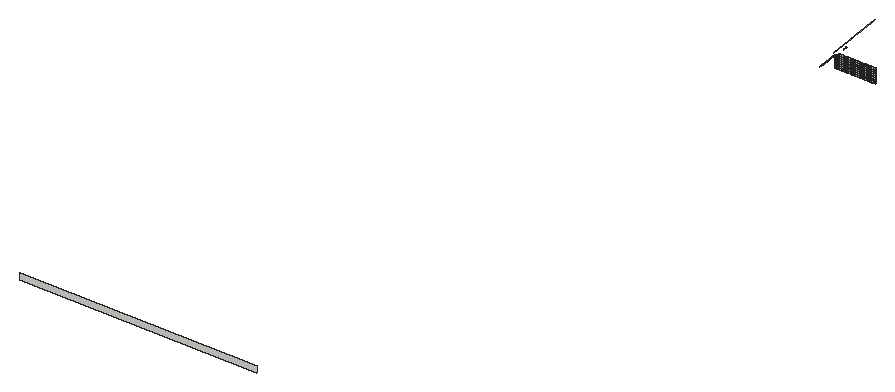
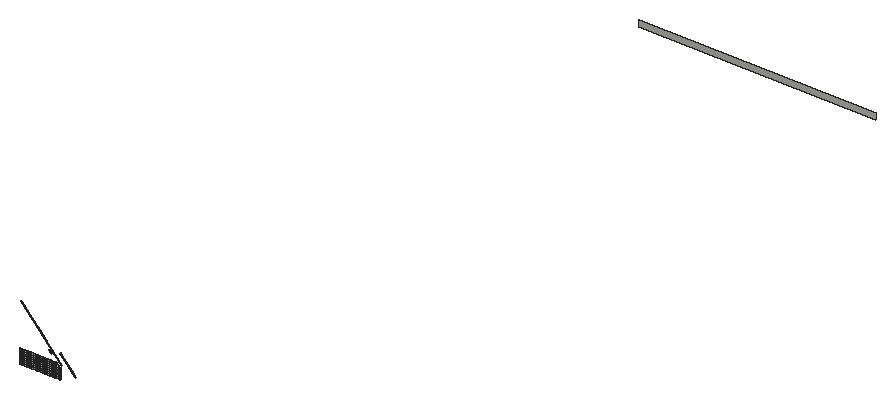
# SketchUp Ruby script. Lengths in inches.
U = 1.inch
M = Sketchup.active_model
def pt(a) = Geom::Point3d.new(a.map { |v| v * U })
def face(e, loops, mat)
  f = e.add_face(loops[0].map { |a| pt(a) })
  loops[1..].each { |l| e.add_face(l.map { |a| pt(a) }).erase! }
  f.material = f.back_material = mat if mat
  f
end
# faces: each face lists its corners as indices into pts; further lists are holes
def faces(e, pts, list, mat = nil) = list.each { |f| face(e, (f[0].is_a?(Array) ? f : [f]).map { |l| l.map { |i| pts[i] } }, mat) }
# xy, xz, yz: faces in a plane at the given z, y or x. An outline is a flat list of corners, or four numbers for a rectangle; further outlines are holes
def ring(l) = l.size == 4 ? [[l[0], l[1]], [l[2], l[1]], [l[2], l[3]], [l[0], l[3]]] : l.each_slice(2).to_a
def flat(e, list, mat, &to3) = list.each { |f| face(e, (f[0].is_a?(Array) ? f : [f]).map { |l| ring(l).map { |u, v| to3.(u, v) } }, mat) }
def xy(e, z, list, mat = nil) = flat(e, list, mat) { |x, y| [x, y, z] }
def xz(e, y, list, mat = nil) = flat(e, list, mat) { |x, z| [x, y, z] }
def yz(e, x, list, mat = nil) = flat(e, list, mat) { |y, z| [x, y, z] }
def lines(e, pts, list) = list.each { |a, b| e.add_line(pt(pts[a]), pt(pts[b])) }
# prism: a flat outline (further loops are holes) pulled along v
def prism(e, loops, v, mat = nil)
  f = face(e, loops, mat); d = Geom::Vector3d.new(v.map { |x| x * U })
  f.pushpull(f.normal.samedirection?(d) ? d.length : -d.length)
end
def box(e, o, s, mat = nil) = prism(e, [[o, [o[0] + s[0], o[1], o[2]], [o[0] + s[0], o[1] + s[1], o[2]], [o[0], o[1] + s[1], o[2]]]], [0, 0, s[2]], mat)
def at(x, y, z, deg = 0) = Geom::Transformation.translation(pt([x, y, z])) * Geom::Transformation.rotation(ORIGIN, Z_AXIS, deg.degrees)
def axes(o, x, y, z) = Geom::Transformation.new([*x, 0, *y, 0, *z, 0, *pt(o).to_a, 1])
def part(name) = M.definitions.add(name)
# library, detail: a bought-in or finely detailed component or shape, given as its bounding box
def library(name, o, s) = part(name).tap { |d| box(d.entities, o, s) }
def detail(e, o, s) = box(e.add_group.entities, o, s)
def put(e, d, t, mat = nil) = e.add_instance(d, t).tap { |i| i.material = mat if mat }
def group(e, t, mat = nil) = e.add_group.tap { |g| g.transformation = t; g.material = mat if mat }.entities
root = M.entities
M.materials.add("[Color M06]").color = [79, 71, 84]
xy(root,305.35,[[951.9,2332.13,954.21,2332.76],[954.8125,2332.13,957.125,2332.76],[957.72,2332.13,960.04,2332.76],[960.64,2332.13,962.95,2332.76],[963.55,2332.13,965.86,2332.76],
  [966.46,2332.13,968.77,2332.76],[969.375,2332.13,971.6875,2332.76],[972.29,2332.13,974.6,2332.76],[975.2,2332.13,977.51,2332.76],[978.11,2332.13,980.42,2332.76],
  [981.02,2332.13,983.33,2332.76],[983.93,2332.13,986.25,2332.76],[986.85,2332.13,989.16,2332.76],[989.76,2332.13,992.07,2332.76],[992.67,2332.13,994.98,2332.76],
  [995.58,2332.13,997.89,2332.76],[998.49,2332.13,1000.81,2332.63],[1001.41,2332.13,1003.72,2332.63],[1004.32,2332.13,1006.63,2332.63],[1007.23,2332.13,1009.54,2332.63],
  [1010.14,2332.13,1012.45,2332.76],[1013.05,2332.13,1015.37,2332.76],[1015.97,2332.13,1018.28,2332.76]])
xy(root,307.67,[[951.9,2332.13,954.21,2332.76],[954.8125,2332.13,957.125,2332.76],[957.72,2332.13,960.04,2332.76],[960.64,2332.13,962.95,2332.76],[963.55,2332.13,965.86,2332.76],
  [966.46,2332.13,968.77,2332.76],[969.375,2332.13,971.6875,2332.76],[972.29,2332.13,974.6,2332.76],[975.2,2332.13,977.51,2332.76],[978.11,2332.13,980.42,2332.76],
  [981.02,2332.13,983.33,2332.76],[983.93,2332.13,986.25,2332.76],[986.85,2332.13,989.16,2332.76],[989.76,2332.13,992.07,2332.76],[992.67,2332.13,994.98,2332.76],
  [995.58,2332.13,997.89,2332.76],[998.49,2332.13,1000.81,2332.63],[1001.41,2332.13,1003.72,2332.63],[1004.32,2332.13,1006.63,2332.63],[1007.23,2332.13,1009.54,2332.63],
  [1010.14,2332.13,1012.45,2332.76],[1013.05,2332.13,1015.37,2332.76],[1015.97,2332.13,1018.28,2332.76]])
xy(root,308.4,[[951.93,2332.13,954.24,2332.76],[954.84,2332.13,957.15,2332.76],[957.75,2332.13,960.07,2332.76],[960.67,2332.13,962.98,2332.76],[963.58,2332.13,965.89,2332.76],
  [966.49,2332.13,968.8,2332.76],[969.4,2332.13,971.71,2332.76],[972.3125,2332.13,974.625,2332.76],[975.23,2332.13,977.54,2332.76],[978.14,2332.13,980.45,2332.76],
  [981.05,2332.13,983.36,2332.76],[983.96,2332.13,986.27,2332.76],[986.875,2332.13,989.1875,2332.76],[989.79,2332.13,992.1,2332.76],[992.7,2332.13,995.01,2332.76],
  [995.61,2332.13,997.92,2332.76],[998.52,2332.13,1000.83,2332.76],[1001.43,2332.13,1003.75,2332.76],[1004.35,2332.13,1006.66,2332.76],[1007.26,2332.13,1009.57,2332.76],
  [1010.17,2332.13,1012.48,2332.76],[1013.08,2332.13,1015.4,2332.76],[1015.99,2332.13,1018.31,2332.76]])
xy(root,310.71,[[951.93,2332.13,954.24,2332.76],[954.84,2332.13,957.15,2332.76],[957.75,2332.13,960.07,2332.76],[960.67,2332.13,962.98,2332.76],[963.58,2332.13,965.89,2332.76],
  [966.49,2332.13,968.8,2332.76],[969.4,2332.13,971.71,2332.76],[972.3125,2332.13,974.625,2332.76],[975.23,2332.13,977.54,2332.76],[978.14,2332.13,980.45,2332.76],
  [981.05,2332.13,983.36,2332.76],[983.96,2332.13,986.27,2332.76],[986.875,2332.13,989.1875,2332.76],[989.79,2332.13,992.1,2332.76],[992.7,2332.13,995.01,2332.76],
  [995.61,2332.13,997.92,2332.76],[998.52,2332.13,1000.83,2332.76],[1001.43,2332.13,1003.75,2332.76],[1004.35,2332.13,1006.66,2332.76],[1007.26,2332.13,1009.57,2332.76],
  [1010.17,2332.13,1012.48,2332.76],[1013.08,2332.13,1015.4,2332.76],[1015.99,2332.13,1018.31,2332.76]])
xy(root,311.21,[[951.93,2332.13,954.24,2332.76],[954.84,2332.13,957.15,2332.76],[957.75,2332.13,960.07,2332.76],[960.67,2332.13,962.98,2332.76],[963.58,2332.13,965.89,2332.76],
  [966.49,2332.13,968.8,2332.76],[969.4,2332.13,971.71,2332.76],[972.3125,2332.13,974.625,2332.76],[975.23,2332.13,977.54,2332.76],[978.14,2332.13,980.45,2332.76],
  [981.05,2332.13,983.36,2332.76],[983.96,2332.13,986.27,2332.76],[986.875,2332.13,989.1875,2332.76],[989.79,2332.13,992.1,2332.76],[992.7,2332.13,995.01,2332.76],
  [995.61,2332.13,997.92,2332.76],[998.52,2332.13,1000.83,2332.76],[1001.43,2332.13,1003.75,2332.76],[1004.35,2332.13,1006.66,2332.76],[1007.26,2332.13,1009.57,2332.76],
  [1010.17,2332.13,1012.48,2332.76],[1013.08,2332.13,1015.4,2332.76],[1015.99,2332.13,1018.31,2332.76]])
xy(root,313.52,[[951.93,2332.13,954.24,2332.76],[954.84,2332.13,957.15,2332.76],[957.75,2332.13,960.07,2332.76],[960.67,2332.13,962.98,2332.76],[963.58,2332.13,965.89,2332.76],
  [966.49,2332.13,968.8,2332.76],[969.4,2332.13,971.71,2332.76],[972.3125,2332.13,974.625,2332.76],[975.23,2332.13,977.54,2332.76],[978.14,2332.13,980.45,2332.76],
  [981.05,2332.13,983.36,2332.76],[983.96,2332.13,986.27,2332.76],[986.875,2332.13,989.1875,2332.76],[989.79,2332.13,992.1,2332.76],[992.7,2332.13,995.01,2332.76],
  [995.61,2332.13,997.92,2332.76],[998.52,2332.13,1000.83,2332.76],[1001.43,2332.13,1003.75,2332.76],[1004.35,2332.13,1006.66,2332.76],[1007.26,2332.13,1009.57,2332.76],
  [1010.17,2332.13,1012.48,2332.76],[1013.08,2332.13,1015.4,2332.76],[1015.99,2332.13,1018.31,2332.76]])
xy(root,314.02,[[951.93,2332.13,954.24,2332.76],[954.84,2332.13,957.15,2332.76],[957.75,2332.13,960.07,2332.76],[960.67,2332.13,962.98,2332.76],[963.58,2332.13,965.89,2332.76],
  [966.49,2332.13,968.8,2332.76],[969.4,2332.13,971.71,2332.76],[972.3125,2332.13,974.625,2332.76],[975.23,2332.13,977.54,2332.76],[978.14,2332.13,980.45,2332.76],
  [981.05,2332.13,983.36,2332.76],[983.96,2332.13,986.27,2332.76],[986.875,2332.13,989.1875,2332.76],[989.79,2332.13,992.1,2332.76],[992.7,2332.13,995.01,2332.76],
  [995.61,2332.13,997.92,2332.76],[998.52,2332.13,1000.83,2332.76],[1001.43,2332.13,1003.75,2332.76],[1004.35,2332.13,1006.66,2332.76],[1007.26,2332.13,1009.57,2332.76],
  [1010.17,2332.13,1012.48,2332.76],[1013.08,2332.13,1015.4,2332.76],[1015.99,2332.13,1018.31,2332.76]])
xy(root,316.34,[[951.93,2332.13,954.24,2332.76],[954.84,2332.13,957.15,2332.76],[957.75,2332.13,960.07,2332.76],[960.67,2332.13,962.98,2332.76],[963.58,2332.13,965.89,2332.76],
  [966.49,2332.13,968.8,2332.76],[969.4,2332.13,971.71,2332.76],[972.3125,2332.13,974.625,2332.76],[975.23,2332.13,977.54,2332.76],[978.14,2332.13,980.45,2332.76],
  [981.05,2332.13,983.36,2332.76],[983.96,2332.13,986.27,2332.76],[986.875,2332.13,989.1875,2332.76],[989.79,2332.13,992.1,2332.76],[992.7,2332.13,995.01,2332.76],
  [995.61,2332.13,997.92,2332.76],[998.52,2332.13,1000.83,2332.76],[1001.43,2332.13,1003.75,2332.76],[1004.35,2332.13,1006.66,2332.76],[1007.26,2332.13,1009.57,2332.76],
  [1010.17,2332.13,1012.48,2332.76],[1013.08,2332.13,1015.4,2332.76],[1015.99,2332.13,1018.31,2332.76]])
xy(root,316.84,[[951.93,2332.13,954.24,2332.76],[954.84,2332.13,957.15,2332.76],[957.75,2332.13,960.07,2332.76],[960.67,2332.13,962.98,2332.76],[963.58,2332.13,965.89,2332.76],
  [966.49,2332.13,968.8,2332.76],[969.4,2332.13,971.71,2332.76],[972.3125,2332.13,974.625,2332.76],[975.23,2332.13,977.54,2332.76],[978.14,2332.13,980.45,2332.76],
  [981.05,2332.13,983.36,2332.76],[983.96,2332.13,986.27,2332.76],[986.875,2332.13,989.1875,2332.76],[989.79,2332.13,992.1,2332.76],[992.7,2332.13,995.01,2332.76],
  [995.61,2332.13,997.92,2332.76],[998.52,2332.13,1000.83,2332.76],[1001.43,2332.13,1003.75,2332.76],[1004.35,2332.13,1006.66,2332.76],[1007.26,2332.13,1009.57,2332.76],
  [1010.17,2332.13,1012.48,2332.76],[1013.08,2332.13,1015.4,2332.76],[1015.99,2332.13,1018.31,2332.76]])
xy(root,319.15,[[951.93,2332.13,954.24,2332.76],[954.84,2332.13,957.15,2332.76],[957.75,2332.13,960.07,2332.76],[960.67,2332.13,962.98,2332.76],[963.58,2332.13,965.89,2332.76],
  [966.49,2332.13,968.8,2332.76],[969.4,2332.13,971.71,2332.76],[972.3125,2332.13,974.625,2332.76],[975.23,2332.13,977.54,2332.76],[978.14,2332.13,980.45,2332.76],
  [981.05,2332.13,983.36,2332.76],[983.96,2332.13,986.27,2332.76],[986.875,2332.13,989.1875,2332.76],[989.79,2332.13,992.1,2332.76],[992.7,2332.13,995.01,2332.76],
  [995.61,2332.13,997.92,2332.76],[998.52,2332.13,1000.83,2332.76],[1001.43,2332.13,1003.75,2332.76],[1004.35,2332.13,1006.66,2332.76],[1007.26,2332.13,1009.57,2332.76],
  [1010.17,2332.13,1012.48,2332.76],[1013.08,2332.13,1015.4,2332.76],[1015.99,2332.13,1018.31,2332.76]])
xy(root,319.65,[[951.93,2332.13,954.24,2332.76],[954.84,2332.13,957.15,2332.76],[957.75,2332.13,960.07,2332.76],[960.67,2332.13,962.98,2332.76],[963.58,2332.13,965.89,2332.76],
  [966.49,2332.13,968.8,2332.76],[969.4,2332.13,971.71,2332.76],[972.3125,2332.13,974.625,2332.76],[975.23,2332.13,977.54,2332.76],[978.14,2332.13,980.45,2332.76],
  [981.05,2332.13,983.36,2332.76],[983.96,2332.13,986.27,2332.76],[986.875,2332.13,989.1875,2332.76],[989.79,2332.13,992.1,2332.76],[992.7,2332.13,995.01,2332.76],
  [995.61,2332.13,997.92,2332.76],[998.52,2332.13,1000.83,2332.76],[1001.43,2332.13,1003.75,2332.76],[1004.35,2332.13,1006.66,2332.7],[1007.26,2332.13,1009.57,2332.7],
  [1010.17,2332.13,1012.48,2332.7],[1013.08,2332.13,1015.4,2332.7],[1015.99,2332.13,1018.31,2332.76]])
xy(root,321.96,[[952.46,2332.13,954.24,2332.76],[954.84,2332.13,957.15,2332.76],[957.75,2332.13,960.07,2332.76],[960.67,2332.13,962.98,2332.76],[963.58,2332.13,965.89,2332.76],
  [966.49,2332.13,968.8,2332.76],[969.4,2332.13,971.71,2332.76],[972.3125,2332.13,974.625,2332.76],[975.23,2332.13,977.54,2332.76],[978.14,2332.13,980.45,2332.76],
  [981.05,2332.13,983.36,2332.76],[983.96,2332.13,986.27,2332.76],[986.875,2332.13,989.1875,2332.76],[989.79,2332.13,992.1,2332.76],[992.7,2332.13,995.01,2332.76],
  [995.61,2332.13,997.92,2332.76],[998.52,2332.13,1000.83,2332.76],[1001.43,2332.13,1003.75,2332.76],[1004.35,2332.13,1006.66,2332.7],[1007.26,2332.13,1009.57,2332.7],
  [1010.17,2332.13,1012.48,2332.7],[1013.08,2332.13,1015.4,2332.7],[1015.99,2332.13,1018.31,2332.76]])
xy(root,322.46,[[954.84,2332.13,957.15,2332.76],[957.75,2332.13,960.07,2332.76],[960.67,2332.13,962.98,2332.76],[963.58,2332.13,965.89,2332.76],[966.49,2332.13,968.8,2332.76],
  [969.4,2332.13,971.71,2332.76],[972.3125,2332.13,974.625,2332.76],[975.23,2332.13,977.54,2332.76],[978.14,2332.13,980.45,2332.76],[981.05,2332.13,983.36,2332.76],
  [983.96,2332.13,986.27,2332.76],[986.875,2332.13,989.1875,2332.76],[989.79,2332.13,992.1,2332.76],[992.7,2332.13,995.01,2332.76],[995.61,2332.13,997.92,2332.76],
  [998.52,2332.13,1000.83,2332.76],[1001.43,2332.13,1003.75,2332.76],[1004.35,2332.13,1006.66,2332.76],[1007.26,2332.13,1009.57,2332.76],[1010.17,2332.13,1012.48,2332.76],
  [1013.08,2332.13,1015.4,2332.76],[1015.99,2332.13,1018.31,2332.76]])
xy(root,324.77,[[955.1,2332.13,957.15,2332.76],[957.75,2332.13,960.07,2332.76],[960.67,2332.13,962.98,2332.76],[963.58,2332.13,965.89,2332.76],[966.49,2332.13,968.8,2332.76],
  [969.4,2332.13,971.71,2332.76],[972.3125,2332.13,974.625,2332.76],[975.23,2332.13,977.54,2332.76],[978.14,2332.13,980.45,2332.76],[981.05,2332.13,983.36,2332.76],
  [983.96,2332.13,986.27,2332.76],[986.875,2332.13,989.1875,2332.76],[989.79,2332.13,992.1,2332.76],[992.7,2332.13,995.01,2332.76],[995.61,2332.13,997.92,2332.76],
  [998.52,2332.13,1000.83,2332.76],[1001.43,2332.13,1003.75,2332.76],[1004.35,2332.13,1006.66,2332.76],[1007.26,2332.13,1009.57,2332.76],[1010.17,2332.13,1012.48,2332.76],
  [1013.08,2332.13,1015.4,2332.76],[1015.99,2332.13,1018.31,2332.76]])
xy(root,325.27,[[957.75,2332.13,960.07,2332.76],[960.67,2332.13,962.98,2332.76],[963.58,2332.13,965.89,2332.76],[966.49,2332.13,968.8,2332.76],[969.4,2332.13,971.71,2332.76],
  [972.3125,2332.13,974.625,2332.76],[975.23,2332.13,977.54,2332.76],[978.14,2332.13,980.45,2332.76],[981.05,2332.13,983.36,2332.76],[983.96,2332.13,986.27,2332.76],
  [986.875,2332.13,989.1875,2332.76],[989.79,2332.13,992.1,2332.76],[992.7,2332.13,995.01,2332.76],[995.61,2332.13,997.92,2332.76],[998.52,2332.13,1000.83,2332.76],
  [1001.43,2332.13,1003.75,2332.76],[1004.35,2332.13,1006.66,2332.76],[1007.26,2332.13,1009.57,2332.76],[1010.17,2332.13,1012.48,2332.76],[1013.08,2332.13,1015.4,2332.76],
  [1015.99,2332.13,1018.31,2332.76]])
xy(root,327.59,[[957.75,2332.13,960.07,2332.76],[960.67,2332.13,962.98,2332.76],[963.58,2332.13,965.89,2332.76],[966.49,2332.13,968.8,2332.76],[972.3125,2332.13,974.625,2332.76],
  [975.23,2332.13,977.54,2332.76],[981.05,2332.13,983.36,2332.76],[983.96,2332.13,986.27,2332.76],[986.875,2332.13,989.1875,2332.76],[992.7,2332.13,995.01,2332.76],
  [995.61,2332.13,997.92,2332.76],[998.52,2332.13,1000.83,2332.76],[1001.43,2332.13,1003.75,2332.76],[1004.35,2332.13,1006.66,2332.76],[1007.26,2332.13,1009.57,2332.76],
  [1010.17,2332.13,1012.48,2332.76],[1013.08,2332.13,1015.4,2332.76],[1015.99,2332.13,1018.31,2332.76]])
xz(root,1201.875,[[522.625,340.125,910.57,350.1875]])
xz(root,2319.18,[[937.8,306.65,940.22,309.22,939.77,309.65,937.35,307.08],[937.35,307.08,939.77,309.65,939.54,309.87,937.12,307.29],[941.1,310.16,943.52,312.73,943.07,313.16,940.64,310.59],[944.4,313.66,946.82,316.23,946.36,316.66,943.94,314.09],[947.7,317.17,950.12,319.74,949.66,320.17,947.24,317.59],
  [951,320.67,953.42,323.24,952.96,323.67,950.54,321.1],[954.29,324.17,956.71,326.75,956.26,327.17,953.84,324.6],[957.59,327.68,960.01,330.25,959.56,330.68,957.14,328.11],[960.89,331.18,963.3125,333.75,962.86,334.18,960.4375,331.61]],"[Color M06]")
xz(root,2332.13,[[954.84,324.5,955.1,324.77,954.84,324.77],[966.49,336.93,968.28,338.84,966.49,338.84],[969.4,340.04,970.91,341.65,969.4,341.65]])
yz(root,951.9,[[2332.13,305.35,2332.76,307.67]])
yz(root,951.93,[[2332.13,308.4,2332.76,310.71],[2332.13,311.21,2332.76,313.52],[2332.13,314.02,2332.76,316.34],[2332.13,316.84,2332.76,319.15],[2332.13,319.65,2332.76,321.39]])
yz(root,954.21,[[2332.13,305.35,2332.76,307.67]])
yz(root,954.24,[[2332.13,308.4,2332.76,310.71],[2332.13,311.21,2332.76,313.52],[2332.13,314.02,2332.76,316.34],[2332.13,316.84,2332.76,319.15],[2332.13,319.65,2332.76,321.96]])
yz(root,954.8125,[[2332.13,305.35,2332.76,307.67]])
yz(root,954.84,[[2332.13,308.4,2332.76,310.71],[2332.13,311.21,2332.76,313.52],[2332.13,314.02,2332.76,316.34],[2332.13,316.84,2332.76,319.15],[2332.13,319.65,2332.76,321.96],
  [2332.13,322.46,2332.76,324.5]])
yz(root,957.125,[[2332.13,305.35,2332.76,307.67]])
yz(root,957.15,[[2332.13,308.4,2332.76,310.71],[2332.13,311.21,2332.76,313.52],[2332.13,314.02,2332.76,316.34],[2332.13,316.84,2332.76,319.15],[2332.13,319.65,2332.76,321.96],
  [2332.13,322.46,2332.76,324.77]])
yz(root,957.72,[[2332.13,305.35,2332.76,307.67]])
yz(root,957.75,[[2332.13,308.4,2332.76,310.71],[2332.13,311.21,2332.76,313.52],[2332.13,314.02,2332.76,316.34],[2332.13,316.84,2332.76,319.15],[2332.13,319.65,2332.76,321.96],
  [2332.13,322.46,2332.76,324.77],[2332.13,325.27,2332.76,327.59]])
yz(root,960.04,[[2332.13,305.35,2332.76,307.67]])
yz(root,960.07,[[2332.13,308.4,2332.76,310.71],[2332.13,311.21,2332.76,313.52],[2332.13,314.02,2332.76,316.34],[2332.13,316.84,2332.76,319.15],[2332.13,319.65,2332.76,321.96],
  [2332.13,322.46,2332.76,324.77],[2332.13,325.27,2332.76,327.59]])
yz(root,960.64,[[2332.13,305.35,2332.76,307.67]])
yz(root,960.67,[[2332.13,308.4,2332.76,310.71],[2332.13,311.21,2332.76,313.52],[2332.13,314.02,2332.76,316.34],[2332.13,316.84,2332.76,319.15],[2332.13,319.65,2332.76,321.96],
  [2332.13,322.46,2332.76,324.77],[2332.13,325.27,2332.76,327.59]])
yz(root,962.95,[[2332.13,305.35,2332.76,307.67]])
yz(root,962.98,[[2332.13,308.4,2332.76,310.71],[2332.13,311.21,2332.76,313.52],[2332.13,314.02,2332.76,316.34],[2332.13,316.84,2332.76,319.15],[2332.13,319.65,2332.76,321.96],
  [2332.13,322.46,2332.76,324.77],[2332.13,325.27,2332.76,327.59]])
yz(root,963.55,[[2332.13,305.35,2332.76,307.67]])
yz(root,963.58,[[2332.13,308.4,2332.76,310.71],[2332.13,311.21,2332.76,313.52],[2332.13,314.02,2332.76,316.34],[2332.13,316.84,2332.76,319.15],[2332.13,319.65,2332.76,321.96],
  [2332.13,322.46,2332.76,324.77],[2332.13,325.27,2332.76,327.59]])
yz(root,965.86,[[2332.13,305.35,2332.76,307.67]])
yz(root,965.89,[[2332.13,308.4,2332.76,310.71],[2332.13,311.21,2332.76,313.52],[2332.13,314.02,2332.76,316.34],[2332.13,316.84,2332.76,319.15],[2332.13,319.65,2332.76,321.96],
  [2332.13,322.46,2332.76,324.77],[2332.13,325.27,2332.76,327.59]])
yz(root,966.46,[[2332.13,305.35,2332.76,307.67]])
yz(root,966.49,[[2332.13,308.4,2332.76,310.71],[2332.13,311.21,2332.76,313.52],[2332.13,314.02,2332.76,316.34],[2332.13,316.84,2332.76,319.15],[2332.13,319.65,2332.76,321.96],
  [2332.13,322.46,2332.76,324.77],[2332.13,325.27,2332.76,327.59]])
yz(root,968.77,[[2332.13,305.35,2332.76,307.67]])
yz(root,968.8,[[2332.13,308.4,2332.76,310.71],[2332.13,311.21,2332.76,313.52],[2332.13,314.02,2332.76,316.34],[2332.13,316.84,2332.76,319.15],[2332.13,319.65,2332.76,321.96],
  [2332.13,322.46,2332.76,324.77],[2332.13,325.27,2332.76,327.59]])
yz(root,969.375,[[2332.13,305.35,2332.76,307.67]])
yz(root,969.4,[[2332.13,308.4,2332.76,310.71],[2332.13,311.21,2332.76,313.52],[2332.13,314.02,2332.76,316.34],[2332.13,316.84,2332.76,319.15],[2332.13,319.65,2332.76,321.96],
  [2332.13,322.46,2332.76,324.77],[2332.13,325.27,2332.76,327.59]])
yz(root,971.6875,[[2332.13,305.35,2332.76,307.67]])
yz(root,971.71,[[2332.13,308.4,2332.76,310.71],[2332.13,311.21,2332.76,313.52],[2332.13,314.02,2332.76,316.34],[2332.13,316.84,2332.76,319.15],[2332.13,319.65,2332.76,321.96],
  [2332.13,322.46,2332.76,324.77],[2332.13,325.27,2332.76,327.59]])
yz(root,972.29,[[2332.13,305.35,2332.76,307.67]])
yz(root,972.3125,[[2332.13,308.4,2332.76,310.71],[2332.13,311.21,2332.76,313.52],[2332.13,314.02,2332.76,316.34],[2332.13,316.84,2332.76,319.15],[2332.13,319.65,2332.76,321.96],
  [2332.13,322.46,2332.76,324.77],[2332.13,325.27,2332.76,327.59]])
yz(root,974.6,[[2332.13,305.35,2332.76,307.67]])
yz(root,974.625,[[2332.13,308.4,2332.76,310.71],[2332.13,311.21,2332.76,313.52],[2332.13,314.02,2332.76,316.34],[2332.13,316.84,2332.76,319.15],[2332.13,319.65,2332.76,321.96],
  [2332.13,322.46,2332.76,324.77],[2332.13,325.27,2332.76,327.59]])
yz(root,975.2,[[2332.13,305.35,2332.76,307.67]])
yz(root,975.23,[[2332.13,308.4,2332.76,310.71],[2332.13,311.21,2332.76,313.52],[2332.13,314.02,2332.76,316.34],[2332.13,316.84,2332.76,319.15],[2332.13,319.65,2332.76,321.96],
  [2332.13,322.46,2332.76,324.77],[2332.13,325.27,2332.76,327.59]])
yz(root,977.51,[[2332.13,305.35,2332.76,307.67]])
yz(root,977.54,[[2332.13,308.4,2332.76,310.71],[2332.13,311.21,2332.76,313.52],[2332.13,314.02,2332.76,316.34],[2332.13,316.84,2332.76,319.15],[2332.13,319.65,2332.76,321.96],
  [2332.13,322.46,2332.76,324.77],[2332.13,325.27,2332.76,327.59]])
yz(root,978.11,[[2332.13,305.35,2332.76,307.67]])
yz(root,978.14,[[2332.13,308.4,2332.76,310.71],[2332.13,311.21,2332.76,313.52],[2332.13,314.02,2332.76,316.34],[2332.13,316.84,2332.76,319.15],[2332.13,319.65,2332.76,321.96],
  [2332.13,322.46,2332.76,324.77],[2332.13,325.27,2332.76,327.59]])
yz(root,980.42,[[2332.13,305.35,2332.76,307.67]])
yz(root,980.45,[[2332.13,308.4,2332.76,310.71],[2332.13,311.21,2332.76,313.52],[2332.13,314.02,2332.76,316.34],[2332.13,316.84,2332.76,319.15],[2332.13,319.65,2332.76,321.96],
  [2332.13,322.46,2332.76,324.77],[2332.13,325.27,2332.76,327.59]])
yz(root,981.02,[[2332.13,305.35,2332.76,307.67]])
yz(root,981.05,[[2332.13,308.4,2332.76,310.71],[2332.13,311.21,2332.76,313.52],[2332.13,314.02,2332.76,316.34],[2332.13,316.84,2332.76,319.15],[2332.13,319.65,2332.76,321.96],
  [2332.13,322.46,2332.76,324.77],[2332.13,325.27,2332.76,327.59]])
yz(root,983.33,[[2332.13,305.35,2332.76,307.67]])
yz(root,983.36,[[2332.13,308.4,2332.76,310.71],[2332.13,311.21,2332.76,313.52],[2332.13,314.02,2332.76,316.34],[2332.13,316.84,2332.76,319.15],[2332.13,319.65,2332.76,321.96],
  [2332.13,322.46,2332.76,324.77],[2332.13,325.27,2332.76,327.59]])
yz(root,983.93,[[2332.13,305.35,2332.76,307.67]])
yz(root,983.96,[[2332.13,308.4,2332.76,310.71],[2332.13,311.21,2332.76,313.52],[2332.13,314.02,2332.76,316.34],[2332.13,316.84,2332.76,319.15],[2332.13,319.65,2332.76,321.96],
  [2332.13,322.46,2332.76,324.77],[2332.13,325.27,2332.76,327.59]])
yz(root,986.25,[[2332.13,305.35,2332.76,307.67]])
yz(root,986.27,[[2332.13,308.4,2332.76,310.71],[2332.13,311.21,2332.76,313.52],[2332.13,314.02,2332.76,316.34],[2332.13,316.84,2332.76,319.15],[2332.13,319.65,2332.76,321.96],
  [2332.13,322.46,2332.76,324.77],[2332.13,325.27,2332.76,327.59]])
yz(root,986.85,[[2332.13,305.35,2332.76,307.67]])
yz(root,986.875,[[2332.13,308.4,2332.76,310.71],[2332.13,311.21,2332.76,313.52],[2332.13,314.02,2332.76,316.34],[2332.13,316.84,2332.76,319.15],[2332.13,319.65,2332.76,321.96],
  [2332.13,322.46,2332.76,324.77],[2332.13,325.27,2332.76,327.59]])
yz(root,989.16,[[2332.13,305.35,2332.76,307.67]])
yz(root,989.1875,[[2332.13,308.4,2332.76,310.71],[2332.13,311.21,2332.76,313.52],[2332.13,314.02,2332.76,316.34],[2332.13,316.84,2332.76,319.15],[2332.13,319.65,2332.76,321.96],
  [2332.13,322.46,2332.76,324.77],[2332.13,325.27,2332.76,327.59]])
yz(root,989.76,[[2332.13,305.35,2332.76,307.67]])
yz(root,989.79,[[2332.13,308.4,2332.76,310.71],[2332.13,311.21,2332.76,313.52],[2332.13,314.02,2332.76,316.34],[2332.13,316.84,2332.76,319.15],[2332.13,319.65,2332.76,321.96],
  [2332.13,322.46,2332.76,324.77],[2332.13,325.27,2332.76,327.59]])
yz(root,992.07,[[2332.13,305.35,2332.76,307.67]])
yz(root,992.1,[[2332.13,308.4,2332.76,310.71],[2332.13,311.21,2332.76,313.52],[2332.13,314.02,2332.76,316.34],[2332.13,316.84,2332.76,319.15],[2332.13,319.65,2332.76,321.96],
  [2332.13,322.46,2332.76,324.77],[2332.13,325.27,2332.76,327.59]])
yz(root,992.67,[[2332.13,305.35,2332.76,307.67]])
yz(root,992.7,[[2332.13,308.4,2332.76,310.71],[2332.13,311.21,2332.76,313.52],[2332.13,314.02,2332.76,316.34],[2332.13,316.84,2332.76,319.15],[2332.13,319.65,2332.76,321.96],
  [2332.13,322.46,2332.76,324.77],[2332.13,325.27,2332.76,327.59]])
yz(root,994.98,[[2332.13,305.35,2332.76,307.67]])
yz(root,995.01,[[2332.13,308.4,2332.76,310.71],[2332.13,311.21,2332.76,313.52],[2332.13,314.02,2332.76,316.34],[2332.13,316.84,2332.76,319.15],[2332.13,319.65,2332.76,321.96],
  [2332.13,322.46,2332.76,324.77],[2332.13,325.27,2332.76,327.59]])
yz(root,995.58,[[2332.13,305.35,2332.76,307.67]])
yz(root,995.61,[[2332.13,308.4,2332.76,310.71],[2332.13,311.21,2332.76,313.52],[2332.13,314.02,2332.76,316.34],[2332.13,316.84,2332.76,319.15],[2332.13,319.65,2332.76,321.96],
  [2332.13,322.46,2332.76,324.77],[2332.13,325.27,2332.76,327.59]])
yz(root,997.89,[[2332.13,305.35,2332.76,307.67]])
yz(root,997.92,[[2332.13,308.4,2332.76,310.71],[2332.13,311.21,2332.76,313.52],[2332.13,314.02,2332.76,316.34],[2332.13,316.84,2332.76,319.15],[2332.13,319.65,2332.76,321.96],
  [2332.13,322.46,2332.76,324.77],[2332.13,325.27,2332.76,327.59]])
yz(root,998.49,[[2332.13,305.35,2332.63,307.67]])
yz(root,998.52,[[2332.13,308.4,2332.76,310.71],[2332.13,311.21,2332.76,313.52],[2332.13,314.02,2332.76,316.34],[2332.13,316.84,2332.76,319.15],[2332.13,319.65,2332.76,321.96],
  [2332.13,322.46,2332.76,324.77],[2332.13,325.27,2332.76,327.59]])
yz(root,1000.81,[[2332.13,305.35,2332.63,307.67]])
yz(root,1000.83,[[2332.13,308.4,2332.76,310.71],[2332.13,311.21,2332.76,313.52],[2332.13,314.02,2332.76,316.34],[2332.13,316.84,2332.76,319.15],[2332.13,319.65,2332.76,321.96],
  [2332.13,322.46,2332.76,324.77],[2332.13,325.27,2332.76,327.59]])
yz(root,1001.41,[[2332.13,305.35,2332.63,307.67]])
yz(root,1001.43,[[2332.13,308.4,2332.76,310.71],[2332.13,311.21,2332.76,313.52],[2332.13,314.02,2332.76,316.34],[2332.13,316.84,2332.76,319.15],[2332.13,319.65,2332.76,321.96],
  [2332.13,322.46,2332.76,324.77],[2332.13,325.27,2332.76,327.59]])
yz(root,1003.72,[[2332.13,305.35,2332.63,307.67]])
yz(root,1003.75,[[2332.13,308.4,2332.76,310.71],[2332.13,311.21,2332.76,313.52],[2332.13,314.02,2332.76,316.34],[2332.13,316.84,2332.76,319.15],[2332.13,319.65,2332.76,321.96],
  [2332.13,322.46,2332.76,324.77],[2332.13,325.27,2332.76,327.59]])
yz(root,1004.32,[[2332.13,305.35,2332.63,307.67]])
yz(root,1004.35,[[2332.13,308.4,2332.76,310.71],[2332.13,311.21,2332.76,313.52],[2332.13,314.02,2332.76,316.34],[2332.13,316.84,2332.76,319.15],[2332.13,319.65,2332.7,321.96],
  [2332.13,322.46,2332.76,324.77],[2332.13,325.27,2332.76,327.59]])
yz(root,1006.63,[[2332.13,305.35,2332.63,307.67]])
yz(root,1006.66,[[2332.13,308.4,2332.76,310.71],[2332.13,311.21,2332.76,313.52],[2332.13,314.02,2332.76,316.34],[2332.13,316.84,2332.76,319.15],[2332.13,319.65,2332.7,321.96],
  [2332.13,322.46,2332.76,324.77],[2332.13,325.27,2332.76,327.59]])
yz(root,1007.23,[[2332.13,305.35,2332.63,307.67]])
yz(root,1007.26,[[2332.13,308.4,2332.76,310.71],[2332.13,311.21,2332.76,313.52],[2332.13,314.02,2332.76,316.34],[2332.13,316.84,2332.76,319.15],[2332.13,319.65,2332.7,321.96],
  [2332.13,322.46,2332.76,324.77],[2332.13,325.27,2332.76,327.59]])
yz(root,1009.54,[[2332.13,305.35,2332.63,307.67]])
yz(root,1009.57,[[2332.13,308.4,2332.76,310.71],[2332.13,311.21,2332.76,313.52],[2332.13,314.02,2332.76,316.34],[2332.13,316.84,2332.76,319.15],[2332.13,319.65,2332.7,321.96],
  [2332.13,322.46,2332.76,324.77],[2332.13,325.27,2332.76,327.59]])
yz(root,1010.14,[[2332.13,305.35,2332.76,307.67]])
yz(root,1010.17,[[2332.13,308.4,2332.76,310.71],[2332.13,311.21,2332.76,313.52],[2332.13,314.02,2332.76,316.34],[2332.13,316.84,2332.76,319.15],[2332.13,319.65,2332.7,321.96],
  [2332.13,322.46,2332.76,324.77],[2332.13,325.27,2332.76,327.59]])
yz(root,1012.45,[[2332.13,305.35,2332.76,307.67]])
yz(root,1012.48,[[2332.13,308.4,2332.76,310.71],[2332.13,311.21,2332.76,313.52],[2332.13,314.02,2332.76,316.34],[2332.13,316.84,2332.76,319.15],[2332.13,319.65,2332.7,321.96],
  [2332.13,322.46,2332.76,324.77],[2332.13,325.27,2332.76,327.59]])
yz(root,1013.05,[[2332.13,305.35,2332.76,307.67]])
yz(root,1013.08,[[2332.13,308.4,2332.76,310.71],[2332.13,311.21,2332.76,313.52],[2332.13,314.02,2332.76,316.34],[2332.13,316.84,2332.76,319.15],[2332.13,319.65,2332.7,321.96],
  [2332.13,322.46,2332.76,324.77],[2332.13,325.27,2332.76,327.59]])
yz(root,1015.37,[[2332.13,305.35,2332.76,307.67]])
yz(root,1015.4,[[2332.13,308.4,2332.76,310.71],[2332.13,311.21,2332.76,313.52],[2332.13,314.02,2332.76,316.34],[2332.13,316.84,2332.76,319.15],[2332.13,319.65,2332.7,321.96],
  [2332.13,322.46,2332.76,324.77],[2332.13,325.27,2332.76,327.59]])
yz(root,1015.97,[[2332.13,305.35,2332.76,307.67]])
yz(root,1015.99,[[2332.13,308.4,2332.76,310.71],[2332.13,311.21,2332.76,313.52],[2332.13,314.02,2332.76,316.34],[2332.13,316.84,2332.76,319.15],[2332.13,319.65,2332.76,321.96],
  [2332.13,322.46,2332.76,324.77],[2332.13,325.27,2332.76,327.59]])
yz(root,1018.28,[[2332.13,305.35,2332.76,307.67]])
yz(root,1018.31,[[2332.13,308.4,2332.76,310.71],[2332.13,311.21,2332.76,313.52],[2332.13,314.02,2332.76,316.34],[2332.13,316.84,2332.76,319.15],[2332.13,319.65,2332.76,321.96],
  [2332.13,322.46,2332.76,324.77],[2332.13,325.27,2332.76,327.59]])
p = [[952.46,2332.13,321.96],[951.93,2332.13,321.39],[951.93,2332.76,321.39],[952.46,2332.76,321.96],[955.1,2332.13,324.77],[954.84,2332.13,324.5],
  [954.84,2332.76,324.5],[955.1,2332.76,324.77],[1011.26,2332.13,391.9],[1016.77,2332.13,397.75],[1016.77,2332.76,397.75],[949.71,2332.76,326.5],
  [949.71,2332.13,326.5],[972.375,2332.13,350.59],[974.55,2332.13,352.9],[975.23,2332.13,353.62],[977.2,2332.13,355.71],[978.14,2332.13,356.71],
  [979.85,2332.13,358.52],[980.32,2332.13,359.02],[980.45,2332.13,359.17],[981.05,2332.13,359.8],[982.49,2332.13,361.34],[982.97,2332.13,361.84],
  [983.36,2332.13,362.26],[983.96,2332.13,362.9],[985.14,2332.13,364.15],[985.61,2332.13,364.65],[986.27,2332.13,365.35],[986.875,2332.13,365.99],
  [987.79,2332.13,366.96],[988.26,2332.13,367.46],[989.1875,2332.13,368.45],[989.79,2332.13,369.08],[990.4375,2332.13,369.77],[990.91,2332.13,370.27],
  [992.1,2332.13,371.54],[992.7,2332.13,372.18],[993.08,2332.13,372.59],[993.55,2332.13,373.09],[995.01,2332.13,374.63],[995.61,2332.13,375.27],
  [995.73,2332.13,375.4],[996.14,2332.13,375.84],[997.92,2332.13,377.73],[998.73,2332.13,378.59],[1000.83,2332.13,380.82],[1001.43,2332.13,381.46],
  [1003.5,2332.13,383.65],[1004.35,2332.13,384.55],[1006.09,2332.13,386.4],[1006.5,2332.13,386.84],[1006.66,2332.13,387.01],[1007.26,2332.13,387.65],
  [1008.67,2332.13,389.15],[1009.09,2332.13,389.59],[1009.57,2332.13,390.1],[1010.17,2332.13,390.74],[972.32,2332.13,347.77],[951.6,2332.13,325.75]]
faces(root,p,[[0,1,2,3],[4,5,6,7],[8,9,10,11,12,13,14,15,16,17,18,19,20,21,22,23,24,25,26,27,28,29,30,31,32,33,34,35,36,37,38,39,40,41,42,43,44,45,46,47,48,49,50,51,52,53,54,55,56,57]])
lines(root,p,[[58,59]])
